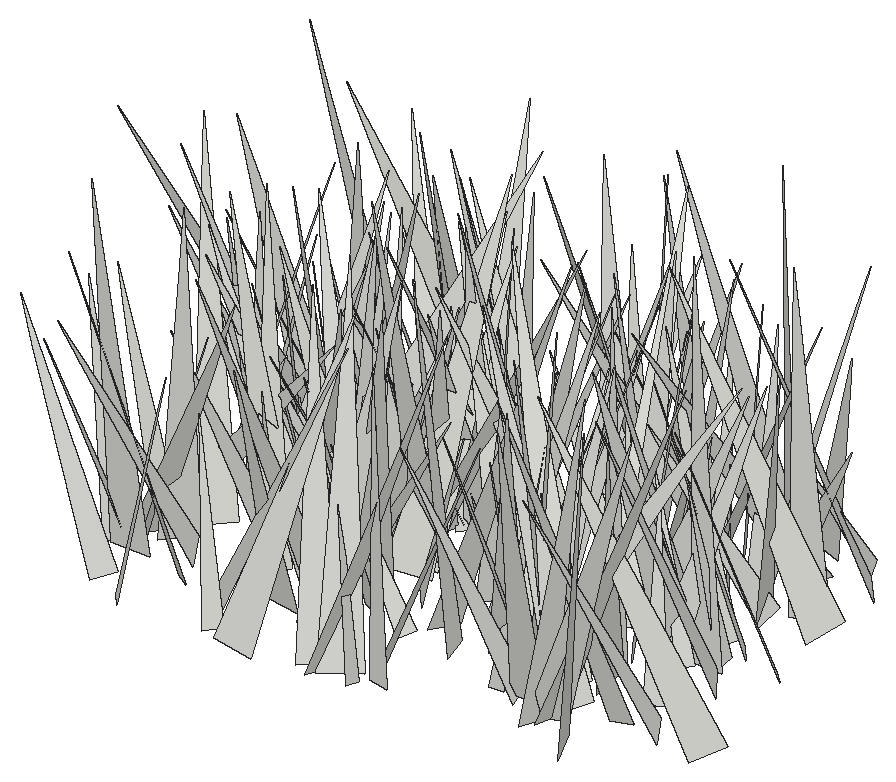
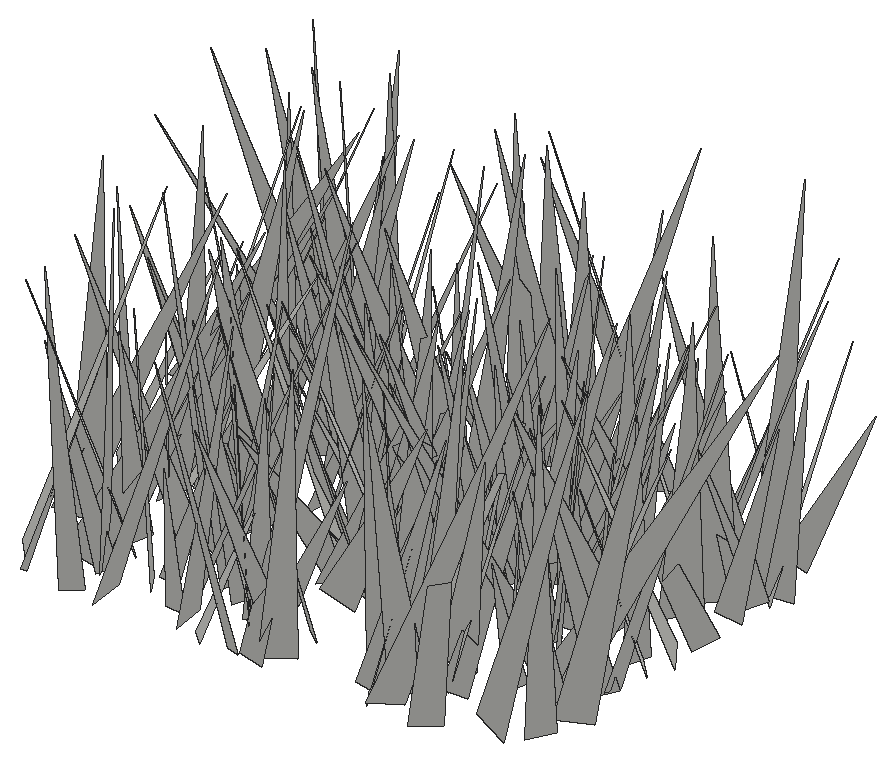
# SketchUp Ruby script. Lengths in inches.
U = 1.inch
M = Sketchup.active_model
def pt(a) = Geom::Point3d.new(a.map { |v| v * U })
def face(e, loops, mat)
  f = e.add_face(loops[0].map { |a| pt(a) })
  loops[1..].each { |l| e.add_face(l.map { |a| pt(a) }).erase! }
  f.material = f.back_material = mat if mat
  f
end
# faces: each face lists its corners as indices into pts; further lists are holes
def faces(e, pts, list, mat = nil) = list.each { |f| face(e, (f[0].is_a?(Array) ? f : [f]).map { |l| l.map { |i| pts[i] } }, mat) }
# xy, xz, yz: faces in a plane at the given z, y or x. An outline is a flat list of corners, or four numbers for a rectangle; further outlines are holes
def ring(l) = l.size == 4 ? [[l[0], l[1]], [l[2], l[1]], [l[2], l[3]], [l[0], l[3]]] : l.each_slice(2).to_a
def flat(e, list, mat, &to3) = list.each { |f| face(e, (f[0].is_a?(Array) ? f : [f]).map { |l| ring(l).map { |u, v| to3.(u, v) } }, mat) }
def xy(e, z, list, mat = nil) = flat(e, list, mat) { |x, y| [x, y, z] }
def xz(e, y, list, mat = nil) = flat(e, list, mat) { |x, z| [x, y, z] }
def yz(e, x, list, mat = nil) = flat(e, list, mat) { |y, z| [x, y, z] }
def lines(e, pts, list) = list.each { |a, b| e.add_line(pt(pts[a]), pt(pts[b])) }
# prism: a flat outline (further loops are holes) pulled along v
def prism(e, loops, v, mat = nil)
  f = face(e, loops, mat); d = Geom::Vector3d.new(v.map { |x| x * U })
  f.pushpull(f.normal.samedirection?(d) ? d.length : -d.length)
end
def box(e, o, s, mat = nil) = prism(e, [[o, [o[0] + s[0], o[1], o[2]], [o[0] + s[0], o[1] + s[1], o[2]], [o[0], o[1] + s[1], o[2]]]], [0, 0, s[2]], mat)
def at(x, y, z, deg = 0) = Geom::Transformation.translation(pt([x, y, z])) * Geom::Transformation.rotation(ORIGIN, Z_AXIS, deg.degrees)
def axes(o, x, y, z) = Geom::Transformation.new([*x, 0, *y, 0, *z, 0, *pt(o).to_a, 1])
def part(name) = M.definitions.add(name)
# library, detail: a bought-in or finely detailed component or shape, given as its bounding box
def library(name, o, s) = part(name).tap { |d| box(d.entities, o, s) }
def detail(e, o, s) = box(e.add_group.entities, o, s)
def put(e, d, t, mat = nil) = e.add_instance(d, t).tap { |i| i.material = mat if mat }
def group(e, t, mat = nil) = e.add_group.tap { |g| g.transformation = t; g.material = mat if mat }.entities
root = M.entities
c1 = part("fur_instance\#9")
p = [[0.8125,0,1.79],[0.67,-0.02,1.48],[0,-0.11,0],[0,0.11,0]]
faces(c1.entities,p,[[0,1,2,3]])
put(root,c1,axes([86.82,379.27,-27.1],[6.37942,2.61315,2.43113],[3.05762,-6.56979,-0.96169],[-1.84118,-1.85616,6.82648]))
put(root,c1,axes([67.4,377.72,-27.1],[3.19373,2.97376,0.94617],[2.91746,-3.32577,0.60507],[-1.10768,-0.18543,4.3217]))
put(root,c1,axes([71.48,378.1875,-27.1],[-3.55756,1.9012,0.49829],[1.88183,3.59228,-0.2708],[0.56709,0.00632,4.02461]))
put(root,c1,axes([72.91,377.54,-27.1],[-0.40245,7.17423,1.83924],[7.10701,0.89237,-1.92572],[2.08393,-1.65784,6.92265]))
put(root,c1,axes([70.46,379.66,-27.1],[6.41393,4.45568,0.74677],[4.39818,-5.86174,-2.80093],[1.0328,-2.70854,7.29015]))
put(root,c1,axes([83.7,381.16,-27.1],[0.50064,-7.21064,0.91051],[-7.21991,-0.3887,0.89157],[0.83387,0.96363,7.17281]))
put(root,c1,axes([77.92,378.21,-27.1],[-4.02809,-0.22088,0.67447],[-0.39433,3.92835,-1.06856],[0.59008,1.11738,3.89005]))
put(root,c1,axes([72.41,381.13,-27.1],[-0.34138,-6.1128,0.75859],[-6.1403,0.39794,0.44341],[0.48829,0.7305,6.10625]))
put(root,c1,axes([67.4,382.32,-27.1],[-5.6995,-3.45113,0.56108],[-3.05969,5.44221,2.39374],[1.69215,-1.78365,6.21808]))
put(root,c1,axes([74.41,381.4375,-27.1],[-0.98604,-7.77609,1.14314],[-7.75331,0.77346,-1.42635],[-1.28859,1.29646,7.70749]))
put(root,c1,axes([78.7,378.72,-27.1],[2.01081,5.29668,2.07869],[5.40677,-2.46554,1.0522],[-1.77275,-1.51176,5.56697]))
put(root,c1,axes([64.83,381.62,-27.1],[-3.71629,-3.62879,0.54604],[-3.4741,3.72939,1.13989],[1.18191,-0.44788,5.0675]))
put(root,c1,axes([65.96,378.8,-27.1],[-1.87407,5.07403,0.37598],[4.58214,1.50899,2.47512],[-2.21159,-1.17322,4.80954]))
put(root,c1,axes([83.11,381.43,-27.1],[-5.60277,-1.40853,0.55452],[-1.25772,5.51462,1.29985],[0.84237,-1.13469,5.62898]))
put(root,c1,axes([88.72,382.41,-27.1],[-5.31145,-3.30369,0.30508],[-3.10318,5.15062,1.7494],[1.17379,-1.33255,6.00546]))
put(root,c1,axes([76.02,378.6,-27.1],[-5.00326,5.02156,1.24961],[5.08502,5.09325,-0.10752],[0.95924,-0.80806,7.08781]))
put(root,c1,axes([65.47,380.93,-27.1],[-0.06707,-7.91469,2.47451],[-8.29222,0.04381,-0.08466],[-0.06773,2.47503,7.91452]))
put(root,c1,axes([76.33,378.13,-27.1],[6.99612,0.8962,1.32294],[0.53893,-6.91662,1.83548],[-1.5043,1.69005,6.81028]))
put(root,c1,axes([77.11,378.53,-27.1],[-4.81371,6.17541,1.55135],[6.27572,4.93015,-0.15223],[1.07597,-1.1279,7.82843]))
put(root,c1,axes([68.33,380.37,-27.1],[-4.54723,-4.75664,0.92618],[-4.80738,4.26788,-1.68375],[-0.61038,1.82216,6.36144]))
put(root,c1,axes([85.05,380.57,-27.1],[5.41416,-4.66063,0.97473],[-4.76032,-5.26587,1.26282],[0.1044,1.59183,7.03135]))
put(root,c1,axes([84.84,380.18,-27.1],[6.67765,-1.57713,2.05629],[-1.75682,-6.93326,0.38749],[-1.90506,0.86558,6.85042]))
put(root,c1,axes([81.29,383.01,-27.1],[1.38948,-7.3294,0.52561],[-7.22169,-1.26322,1.47599],[1.35779,0.7818,7.31247]))
put(root,c1,axes([82.22,383.17,-27.1],[-4.28945,-4.51982,0.83876],[-4.25056,4.33652,1.63064],[1.75072,-0.54543,6.01408]))
put(root,c1,axes([74.53,380.42,-27.1],[-0.74897,7.24815,2.93985],[7.55595,1.43371,-1.60981],[2.0214,-2.6736,7.1067]))
put(root,c1,axes([87.3,382.05,-27.1],[-2.01567,-6.30283,1.43527],[-6.28052,1.55369,-1.99742],[-1.52993,1.92587,6.30864]))
put(root,c1,axes([75.15,382.85,-27.1],[-2.33347,-4.94017,0.88075],[-4.99474,2.38012,0.11709],[0.48332,0.74554,5.4623]))
put(root,c1,axes([64.7,381.16,-27.1],[-2.06507,4.56305,1.47225],[4.79287,1.92061,0.77009],[-0.13147,-1.65628,4.94903]))
put(root,c1,axes([85.13,380.65,-27.1],[7.79072,-0.23447,0.87822],[-0.35324,-7.76347,1.06082],[-0.83754,1.09323,7.72172]))
put(root,c1,axes([72.3125,383.0625,-27.1],[-4.28655,1.17606,1.86698],[1.8295,4.17484,1.57066],[1.23356,-2.10497,4.15821]))
put(root,c1,axes([74.13,383.9,-27.1],[5.44226,-5.9088,0.26751],[-5.91243,-5.44486,0.01623],[-0.16928,0.20777,8.03317]))
put(root,c1,axes([91.21,382.15,-27.1],[-4.16636,5.9481,1.52453],[5.74666,3.12806,3.50054],[-2.16332,-3.14611,6.36276]))
put(root,c1,axes([65.1,382.26,-27.1],[5.86888,-2.59714,0.14419],[-2.59865,-5.83866,0.60558],[0.11385,0.61201,6.38922]))
put(root,c1,axes([85.16,384.0625,-27.1],[6.59264,-0.88288,1.14982],[-0.53637,-6.4595,-1.88457],[-1.3468,-1.74924,6.37893]))
put(root,c1,axes([85.06,381.23,-27.1],[-4.32916,0.66549,1.27706],[0.40908,4.44763,-0.93094],[1.38073,0.76884,4.27993]))
put(root,c1,axes([66.33,382.7,-27.1],[-4.86484,4.13925,3.64162],[4.78109,5.5858,0.03796],[2.74517,-2.39309,6.38738]))
put(root,c1,axes([84.28,381.98,-27.1],[-5.98871,-2.33617,1.80164],[-2.60473,6.10133,-0.74665],[1.38529,1.37273,6.38474]))
put(root,c1,axes([77.84,380.1,-27.1],[3.89032,1.8987,0.46131],[1.51623,-3.58179,1.95558],[-1.23244,1.58688,3.86204]))
put(root,c1,axes([85.3125,381.73,-27.1],[-7.32829,2.58062,0.59876],[2.60966,7.33524,0.32553],[0.45582,-0.50666,7.76257]))
put(root,c1,axes([82.47,382.88,-27.1],[5.33637,4.77614,2.80857],[5.34994,-5.45601,-0.88678],[-1.44141,-2.56842,7.10647]))
put(root,c1,axes([79.25,382.46,-27.1],[-6.68963,-2.36331,2.10659],[-2.62997,6.88987,-0.62215],[1.76244,1.31094,7.06748]))
put(root,c1,axes([89.59,383.45,-27.1],[-6.11827,1.22354,0.04324],[1.20265,5.96505,1.37981],[-0.22923,-1.36132,6.08493]))
put(root,c1,axes([77.21,382.24,-27.1],[-1.66623,3.3763,0.05798],[2.90925,1.40249,1.93607],[-1.71436,-0.9015,3.22914]))
put(root,c1,axes([65.49,381.56,-27.1],[3.79033,1.52401,0.8214],[1.29616,-3.80865,1.0854],[-1.14773,0.73179,3.93842]))
put(root,c1,axes([81.27,383.68,-27.1],[-2.39364,-3.13142,1.17859],[-3.27618,2.48779,-0.04385],[0.67935,0.9641,3.94124]))
put(root,c1,axes([68.75,384.91,-27.1],[0.69444,-4.60057,1.02449],[-4.36557,-1.0182,-1.61314],[-1.77671,0.70364,4.36409]))
put(root,c1,axes([82.21,381.15,-27.1],[2.45384,5.3856,0.3895],[5.06414,-2.44383,1.88676],[-1.87372,0.44803,5.60947]))
put(root,c1,axes([83.4375,383.82,-27.1],[-3.37227,-0.8607,0.92289],[-0.91034,3.4828,-0.07828],[0.87397,0.30665,3.4795]))
put(root,c1,axes([88.16,386.44,-27.1],[-5.39374,-4.42373,0.73063],[-4.15874,5.36317,1.77113],[1.67573,-0.92879,6.74722]))
put(root,c1,axes([75.81,384.79,-27.1],[3.73133,2.74864,1.27928],[3.02044,-3.19509,-1.94493],[0.26177,-2.31318,4.20655]))
put(root,c1,axes([65.27,383.4,-27.1],[-1.60239,4.56784,1.22355],[4.62571,1.24567,1.40748],[-0.98238,-1.58525,4.63161]))
put(root,c1,axes([69.11,384.76,-27.1],[3.4639,-0.21189,1.20284],[0.06017,-3.58323,-0.80448],[-1.21988,-0.7784,3.37584]))
put(root,c1,axes([70.13,383.94,-27.1],[-6.35948,3.06032,1.72749],[3.24757,6.48259,0.47123],[1.34279,-1.18457,7.04176]))
put(root,c1,axes([82.43,382.77,-27.1],[3.56611,7.00423,0.23479],[6.50816,-3.2121,-3.02618],[2.59966,-1.56674,7.25387]))
put(root,c1,axes([87.46,383.78,-27.1],[-1.55614,3.71904,0.91385],[3.82438,1.56093,0.15988],[0.20123,-0.90564,4.0283]))
put(root,c1,axes([70.16,383.97,-27.1],[-2.19401,4.08598,0.64459],[3.98986,1.89782,1.55038],[-1.09165,-1.27572,4.37096]))
put(root,c1,axes([73.15,384.03,-27.1],[4.12414,-1.44643,0.07491],[-1.4095,-3.95608,1.21201],[0.33327,1.1677,4.19901]))
put(root,c1,axes([84,383.02,-27.1],[-6.13421,5.52562,0.24546],[5.52788,6.11218,0.5523],[-0.18784,-0.57446,8.23747]))
put(root,c1,axes([70.47,382.9,-27.1],[-6.55915,2.85076,0.80174],[2.70921,6.56329,-1.17278],[1.19574,0.76707,7.05506]))
put(root,c1,axes([82.21,383.78,-27.1],[-0.35457,5.93898,1.63328],[6.05839,0.63143,-0.98081],[1.11129,-1.54746,5.86815]))
put(root,c1,axes([73.56,386,-27.1],[-2.21504,-4.22644,0.02495],[-4.06696,2.12371,-1.31133],[-1.15036,0.62998,4.58799]))
put(root,c1,axes([64.6875,385.44,-27.1],[2.58062,-5.27777,0.62862],[-4.46822,-1.77579,3.43383],[2.87837,1.97518,4.76689]))
put(root,c1,axes([69.66,386.86,-27.1],[6.23542,-1.61716,0.46655],[-1.48447,-6.12774,-1.40019],[-0.79324,-1.24458,6.2877]))
put(root,c1,axes([85.625,387.6,-27.1],[5.45366,-4.66647,1.60556],[-4.21255,-5.64853,-2.10822],[-2.57063,-0.64365,6.86103]))
put(root,c1,axes([70.11,385.39,-27.1],[-5.34119,3.3335,0.99515],[3.47843,5.14626,1.43085],[0.05516,-1.74201,6.13133]))
put(root,c1,axes([79.4375,384.82,-27.1],[2.86437,6.58912,2.04567],[6.83224,-2.40073,-1.83379],[0.96006,-2.57407,6.94682]))
put(root,c1,axes([77.86,383.58,-27.1],[7.57177,-0.43303,1.80554],[-0.88332,-7.50835,1.90355],[-1.63317,2.05334,7.34137]))
put(root,c1,axes([81.09,383.83,-27.1],[-3.67286,3.55796,0.5072],[3.52102,3.70767,-0.51167],[0.72023,0.01818,5.08794]))
put(root,c1,axes([74.72,386.87,-27.1],[-1.19832,-8.06423,2.00487],[-8.30399,1.23724,0.01324],[0.30817,1.98109,8.15276]))
put(root,c1,axes([78.06,386.12,-27.1],[3.7544,-3.60472,1.46029],[-3.77286,-3.86843,0.15082],[-0.94444,1.12393,5.20257]))
put(root,c1,axes([84.68,385,-27.1],[1.78909,6.44129,2.50482],[6.73985,-2.19865,0.83993],[-1.52927,-2.15428,6.63216]))
put(root,c1,axes([72.03,386.16,-27.1],[-5.02266,3.34128,1.54054],[3.64584,4.87057,1.32283],[0.49523,-1.96924,5.88569]))
put(root,c1,axes([69.45,387.61,-27.1],[3.15853,-4.87453,2.05329],[-4.28659,-3.76007,-2.33247],[-3.09874,0.23284,5.31949]))
put(root,c1,axes([66.7,384.33,-27.1],[-6.24341,4.5177,1.05822],[4.50521,6.32678,-0.4296],[1.11019,-0.26807,7.69449]))
put(root,c1,axes([69.52,386.68,-27.1],[-3.89073,-3.2521,0.98713],[-3.3181,3.95947,-0.03367],[0.73538,0.65937,5.07078]))
put(root,c1,axes([72.9,385.89,-27.1],[4.30722,-1.10997,0.82887],[-1.21703,-4.32511,0.53238],[-0.66174,0.72977,4.41597]))
put(root,c1,axes([70.14,386.71,-27.1],[-7.66892,-1.90839,0.15613],[-1.91216,7.66661,-0.21311],[0.09999,0.24454,7.89993]))
put(root,c1,axes([66.61,387.25,-27.1],[-5.67591,-0.59927,2.29984],[-0.30227,6.08824,0.84044],[2.35734,-0.66225,5.64524]))
put(root,c1,axes([81.92,386.47,-27.1],[-5.15429,0.32159,0.0951],[0.32057,5.15491,-0.05731],[0.09848,0.05128,5.164]))
put(root,c1,axes([80.93,387,-27.1],[-7.3033,-3.33888,1.09507],[-3.45877,7.27632,-0.88176],[0.61989,1.26191,7.98178]))
put(root,c1,axes([69.2,388.52,-27.1],[6.14406,2.36607,3.59044],[3.36505,-6.54408,-1.44586],[-2.67694,-2.79567,6.42319]))
put(root,c1,axes([73.43,388.87,-27.1],[5.23311,-3.59302,0.50013],[-3.53385,-5.24745,-0.7222],[-0.81967,-0.31597,6.30664]))
put(root,c1,axes([71.98,385.66,-27.1],[-5.31881,4.24046,0.31909],[4.24772,5.322,0.07866],[0.20039,-0.26047,6.80184]))
put(root,c1,axes([72.93,384.17,-27.1],[1.87355,6.48838,0.26131],[6.01197,-1.83596,2.48253],[-2.45429,0.45575,6.28063]))
put(root,c1,axes([87.48,387.77,-27.1],[-3.67755,-0.2078,1.11626],[-0.0694,3.8179,0.48208],[1.13331,-0.4405,3.65173]))
put(root,c1,axes([71.16,386.72,-27.1],[1.59622,5.71911,2.00108],[6.0184,-1.73595,0.16062],[-0.70101,-1.88115,5.93551]))
put(root,c1,axes([84.43,386.23,-27.1],[5.20843,4.28763,1.83578],[4.29945,-5.48037,0.60158],[-1.80791,-0.68076,6.71935]))
put(root,c1,axes([89.64,388.16,-27.1],[-3.75562,-3.58045,0.3486],[-3.58145,3.67402,-0.84892],[-0.33818,0.85312,5.11895]))
put(root,c1,axes([65.1875,390.17,-27.1],[-6.16239,-2.08969,1.53365],[-1.42213,6.03269,2.50561],[2.16712,-1.98337,6.00531]))
put(root,c1,axes([79.35,385.98,-27.1],[3.38601,2.0667,0.33408],[1.88033,-3.28152,1.24252],[-0.92044,0.89903,3.76728]))
put(root,c1,axes([86.52,386.68,-27.1],[-0.98772,3.5916,0.11089],[3.35733,0.88143,1.35606],[-1.28071,-0.45933,3.46934]))
put(root,c1,axes([74.43,385.77,-27.1],[-3.17908,7.18759,1.82609],[7.05927,3.54175,-1.65087],[2.27218,-0.9472,7.68392]))
put(root,c1,axes([87.15,387.12,-27.1],[1.25442,7.48082,2.76942],[7.81491,-1.71475,1.09211],[-1.59984,-2.51056,7.50623]))
put(root,c1,axes([72.58,387.64,-27.1],[4.97792,-1.2009,1.19397],[-1.36113,-5.04298,0.6026],[-1.0075,0.87956,5.08515]))
put(root,c1,axes([85.42,387,-27.1],[0.44188,5.84269,1.52194],[5.83939,-0.02571,-1.59672],[1.53457,-1.58458,5.63763]))
put(root,c1,axes([74.9,389.9375,-27.1],[1.62052,-5.44249,0.65001],[-5.43307,-1.68456,-0.55967],[-0.72449,0.45919,5.65098]))
put(root,c1,axes([87.62,388.77,-27.1],[-4.41159,-3.54695,0.73212],[-3.61607,4.3782,-0.57829],[0.20221,0.91078,5.63104]))
put(root,c1,axes([73.36,385.91,-27.1],[1.09357,6.43106,0.77169],[6.11568,-1.28298,2.02542],[-2.13365,-0.38127,6.20097]))
put(root,c1,axes([72.23,389.6,-27.1],[-3.11173,-3.4795,0.92655],[-3.33661,3.24675,0.98692],[1.3537,0.0043,4.56244]))
put(root,c1,axes([65.85,387.97,-27.1],[-4.75498,1.70819,1.94206],[1.76287,5.11453,-0.18234],[1.89256,-0.47231,5.04921]))
put(root,c1,axes([73.33,390.19,-27.1],[-3.18461,-4.17271,0.10236],[-4.17132,3.18622,0.10881],[0.1486,0.01532,5.24799]))
put(root,c1,axes([75.9,390.62,-27.1],[-1.54524,-6.7658,0.51217],[-6.71547,1.44992,-1.10738],[-0.96994,0.74015,6.85109]))
put(root,c1,axes([77.31,388.77,-27.1],[6.16664,-2.56617,1.31423],[-2.70082,-6.22755,0.51287],[-1.00896,0.98602,6.65955]))
put(root,c1,axes([69.11,389.09,-27.1],[7.358,-0.55238,1.16955],[-0.51092,-7.44716,-0.30295],[-1.18825,-0.21839,7.37248]))
put(root,c1,axes([73.91,387.28,-27.1],[7.28902,-0.71217,0.57332],[-0.83779,-7.04721,1.89755],[-0.36604,1.94818,7.07364]))
put(root,c1,axes([67.05,390.84,-27.1],[-1.39061,-8.04384,0.83594],[-7.45661,0.94696,-3.29214],[-3.13068,1.31752,7.46987]))
put(root,c1,axes([74.43,386.53,-27.1],[-1.14169,6.19263,0.48775],[6.13199,1.20279,-0.91762],[0.99261,-0.30768,6.22978]))
put(root,c1,axes([67.7,390.29,-27.1],[-3.39488,-3.98848,1.56761],[-3.7052,3.73666,1.48306],[2.15333,0.14147,5.02331]))
put(root,c1,axes([66.82,389.33,-27.1],[-2.76326,-3.0585,1.38467],[-3.15346,2.97986,0.28892],[1.15213,0.82059,4.11176]))
put(root,c1,axes([86.87,387.49,-27.1],[-6.97142,-3.26118,0.0354],[-2.96258,6.29742,-3.28677],[-1.3637,2.99072,6.9594]))
put(root,c1,axes([78.18,390.34,-27.1],[-6.07615,0.58264,0.90457],[0.83184,5.83413,1.82981],[0.68247,-1.92372,5.8233]))
put(root,c1,axes([77.59,387.75,-27.1],[-3.01404,5.97197,0.86388],[5.95256,2.78442,1.51964],[-0.98886,-1.44144,6.51457]))
put(root,c1,axes([65,386.75,-27.1],[5.18703,3.91751,0.7095],[3.72248,-5.18551,1.41748],[-1.41191,0.72053,6.34373]))
put(root,c1,axes([74.58,390.03,-27.1],[2.81734,-6.20209,1.85033],[-6.41792,-2.93797,-0.07572],[-0.83667,1.65211,6.81158]))
put(root,c1,axes([77.36,390.13,-27.1],[-4.25466,-1.2014,1.34721],[-0.93808,4.41863,0.97784],[1.54219,-0.62673,4.31153]))
put(root,c1,axes([76.05,389.45,-27.1],[-1.30466,-3.28465,1.2487],[-3.51229,1.2605,-0.354],[0.10971,1.29326,3.5165]))
put(root,c1,axes([77.03,387.84,-27.1],[4.58247,4.01128,0.43645],[4.00699,-4.60163,0.22113],[-0.47421,-0.12046,6.08609]))
put(root,c1,axes([79.41,387.74,-27.1],[-0.73079,4.32054,0.1844],[4.30671,0.74406,-0.36572],[0.39156,-0.12013,4.36662]))
put(root,c1,axes([86.65,391.39,-27.1],[-4.86866,0.51762,1.11395],[0.97098,4.41082,2.19421],[0.75234,-2.34296,4.3769]))
put(root,c1,axes([78.57,388.875,-27.1],[5.68273,3.19615,0.64935],[3.24559,-5.67036,-0.49352],[-0.32122,-0.74969,6.50117]))
put(root,c1,axes([82.98,389.33,-27.1],[2.29321,-4.71361,1.70331],[-4.8602,-1.63403,2.02152],[1.22385,2.34308,4.83635]))
put(root,c1,axes([67.81,386.84,-27.1],[-5.19171,3.73852,1.55221],[3.028,5.26206,-2.54592],[2.68647,1.29382,5.8693]))
put(root,c1,axes([86.6,388.86,-27.1],[-5.80582,1.67481,0.45332],[1.66732,5.82342,-0.1609],[0.48013,0.02943,6.04042]))
put(root,c1,axes([75.09,389.45,-27.1],[-3.69691,-1.68274,0.52652],[-1.75981,3.59718,-0.85985],[0.10916,1.00233,3.96981]))
put(root,c1,axes([65.32,388.14,-27.1],[3.04107,3.48011,0.59696],[3.3547,-3.09349,0.94446],[-1.10161,0.1866,4.52408]))
put(root,c1,axes([65.24,390.52,-27.1],[2.87453,-4.20489,0.68169],[-4.14129,-2.56592,1.63539],[0.99777,1.46412,4.82385]))
put(root,c1,axes([86.32,391.51,-27.1],[6.10646,0.88523,1.50787],[1.27518,-6.00248,-1.64024],[-1.19633,-1.87958,5.94829]))
put(root,c1,axes([82.58,388.76,-27.1],[-5.70861,3.53079,2.01517],[3.32922,6.05385,-1.17592],[2.33318,0.00055,6.60847]))
put(root,c1,axes([68.99,391.07,-27.1],[-4.42725,-2.60663,1.07476],[-2.66002,4.52485,0.01676],[0.93485,0.53053,5.13759]))
put(root,c1,axes([74.09,389.63,-27.1],[-3.60805,2.068,0.36238],[2.05277,3.62596,-0.25393],[0.44056,0.04128,4.15092]))
put(root,c1,axes([66.03,392.33,-27.1],[-3.26059,-4.43586,0.10579],[-4.43536,3.26207,0.0775],[0.12511,0.03932,5.50476]))
put(root,c1,axes([82.9,389.68,-27.1],[-6.0397,-1.24718,1.08354],[-1.47294,5.92489,-1.39057],[0.74831,1.59618,6.00831]))
put(root,c1,axes([69.53,393.93,-27.1],[4.70734,-3.12135,0.14145],[-2.64852,-4.12178,-2.81392],[-1.65776,-2.27815,4.89732]))
put(root,c1,axes([72.9,388.29,-27.1],[-1.71935,6.00909,0.23442],[5.94835,1.73522,-0.85232],[0.8839,0.01135,6.19184]))
put(root,c1,axes([88.93,391.78,-27.1],[-7.28796,2.50197,0.93453],[2.66483,6.99355,2.0583],[0.17855,-2.25345,7.42547]))
put(root,c1,axes([82.76,387.55,-27.1],[-4.41357,6.91206,0.00056],[6.86097,4.38103,-0.99489],[0.83882,0.53496,8.14041]))
put(root,c1,axes([82.66,391.3,-27.1],[-2.78435,-5.66723,3.39056],[-5.97834,3.72634,1.319],[2.80584,2.3158,6.17497]))
put(root,c1,axes([75.77,390.88,-27.1],[4.35224,4.23695,0.82253],[4.28263,-4.09432,-1.57033],[0.53605,-1.68972,5.86752]))
put(root,c1,axes([64.83,392.85,-27.1],[4.91943,-4.73173,2.30235],[-4.40019,-5.42749,-1.75256],[-2.8859,0.2095,6.59686]))
put(root,c1,axes([86.2,394.54,-27.1],[2.18391,-6.70079,0.42323],[-6.08063,-2.16263,-2.86325],[-2.84706,-0.52116,6.43986]))
put(root,c1,axes([84.6,391.5625,-27.1],[2.87799,2.64757,1.74089],[2.94858,-3.09885,-0.16173],[-1.16026,-1.30792,3.90721]))
put(root,c1,axes([80.87,394.9375,-27.1],[-6.78403,-3.28205,0.63683],[-2.89291,6.48484,2.60352],[1.67585,-2.09175,7.07224]))
put(root,c1,axes([87.93,392.14,-27.1],[1.68119,-6.78383,2.85706],[-7.30642,-1.89388,-0.19753],[-0.89411,2.72073,6.98625]))
put(root,c1,axes([83.46,391.49,-27.1],[6.47298,0.85818,0.33872],[0.84258,-6.4766,0.30739],[-0.37587,0.26066,6.52238]))
put(root,c1,axes([67.67,393.18,-27.1],[3.15596,1.30372,1.61225],[1.82364,-3.14251,-1.02861],[-0.98659,-1.6383,3.25603]))
put(root,c1,axes([80.8125,392.86,-27.1],[3.7872,-0.0255,0.26622],[0.02172,-3.73751,-0.66706],[-0.26655,-0.66693,3.72808]))
put(root,c1,axes([70.03,393.65,-27.1],[-3.79874,-3.55526,0.6962],[-3.51199,3.8615,0.55657],[0.88909,0.06302,5.17306]))
put(root,c1,axes([79.05,388.97,-27.1],[-4.90566,2.32822,0.51514],[1.6552,4.17303,-3.098],[1.71648,2.62995,4.45965]))
put(root,c1,axes([68.17,390.375,-27.1],[0.84349,7.5995,0.98427],[7.14395,-0.42161,-2.86687],[2.77222,-1.22577,7.08837]))
put(root,c1,axes([82.73,393.87,-27.1],[0.53786,-3.60504,0.14249],[-3.55289,-0.5543,-0.6129],[-0.62738,0.04841,3.59304]))
put(root,c1,axes([78.45,392.29,-27.1],[-1.80359,3.13263,0.44398],[3.00697,1.53819,1.36218],[-0.98418,-1.04117,3.34825]))
put(root,c1,axes([73.66,391.81,-27.1],[0.00503,4.167,0.7042],[4.17874,-0.11,0.62111],[-0.63075,-0.69557,4.12045]))
put(root,c1,axes([72.98,392.79,-27.1],[4.34542,2.75412,2.00138],[2.98226,-4.64462,-0.0836],[-1.6422,-1.14703,5.14401]))
put(root,c1,axes([77.11,391.17,-27.1],[-1.95645,6.57203,0.15793],[5.85701,1.66776,3.15567],[-2.98529,-1.03499,6.08778]))
put(root,c1,axes([79.6875,393.24,-27.1],[5.0608,-1.8582,0.79428],[-1.91101,-5.09708,0.2516],[-0.65714,0.51221,5.38529]))
put(root,c1,axes([78.59,394.21,-27.1],[4.23217,0.79223,1.75299],[1.35483,-4.23497,-1.35698],[-1.36567,-1.74623,4.08626]))
put(root,c1,axes([69.9375,394.875,-27.1],[-3.5221,-6.63629,1.77015],[-6.5539,3.84233,1.36448],[2.0543,0.8804,7.38808]))
put(root,c1,axes([66.11,392.15,-27.1],[0.58745,4.61701,1.14714],[4.75417,-0.52722,-0.31264],[0.17496,-1.17604,4.64372]))
put(root,c1,axes([88.25,395.33,-27.1],[-5.65228,-5.31186,0.60473],[-5.29476,5.68375,0.43618],[0.73959,0.09466,7.74428]))
put(root,c1,axes([85.47,392.18,-27.1],[-4.49774,2.41965,1.22715],[2.26445,4.65664,-0.88215],[1.49428,0.22634,5.03052]))
put(root,c1,axes([65.13,394.39,-27.1],[5.79339,-2.08626,1.56673],[-1.97661,-6.00002,-0.68061],[-1.70297,-0.13319,6.11985]))
put(root,c1,axes([76.8,396.55,-27.1],[-3.41876,-7.6362,0.72671],[-7.48826,3.49493,1.49637],[1.66304,0.03883,8.23167]))
put(root,c1,axes([84.99,394.63,-27.1],[1.43751,-4.12245,0.23292],[-3.7226,-1.18725,1.96162],[1.78636,0.84328,3.90039]))
put(root,c1,axes([71,396.04,-27.1],[-7.92224,1.63819,2.17065],[2.33717,7.51957,2.85498],[1.39032,-3.306,7.56932]))
put(root,c1,axes([68.85,396.39,-27.1],[6.56004,-2.8558,0.90961],[-2.50702,-6.42798,-2.10074],[-1.6425,-1.59457,6.83935]))
put(root,c1,axes([68.02,392.2,-27.1],[-3.33951,2.40161,0.05247],[2.31618,3.24301,-1.02031],[0.63702,0.79874,3.98485]))
put(root,c1,axes([72.96,393.85,-27.1],[5.47635,-0.94494,2.24683],[-1.1073,-5.8869,0.22307],[-2.17142,0.61884,5.55279]))
put(root,c1,axes([76.0625,393.84,-27.1],[4.67492,4.49227,1.13099],[4.6277,-4.45606,-1.42912],[0.20972,-1.8104,6.324]))
put(root,c1,axes([70.71,392.2,-27.1],[-2.20757,6.36235,0.08993],[6.1827,2.12231,1.62203],[-1.50393,-0.61421,6.5362]))
put(root,c1,axes([83.06,394.42,-27.1],[4.36466,2.86173,1.95624],[3.18404,-4.55325,-0.44325],[-1.3705,-1.46462,5.20032]))
put(root,c1,axes([87.36,396.49,-27.1],[-3.37323,-1.69913,0.74168],[-1.13548,3.11072,1.96213],[1.46554,-1.50074,3.22735]))
put(root,c1,axes([85.39,392.65,-27.1],[4.30738,5.01035,0.65824],[4.94004,-4.35705,0.83813],[-1.06435,0.05398,6.55397]))
put(root,c1,axes([66.9375,395.06,-27.1],[-2.69995,-7.06667,2.40673],[-7.39529,2.18224,-1.88876],[-1.01973,2.88442,7.32531]))
put(root,c1,axes([78.63,394.4375,-27.1],[-4.89725,-3.9807,3.26033],[-4.56553,5.43754,-0.21877],[2.37312,2.24631,6.30723]))
put(root,c1,axes([85.51,394.09,-27.1],[-6.98093,-2.98191,2.95578],[-3.56155,7.24267,-1.10492],[2.22346,2.23913,7.51028]))
put(root,c1,axes([78.3,394.26,-27.1],[-1.55203,4.86816,1.43833],[5.0761,1.479,0.47157],[-0.03172,-1.51332,5.08777]))
put(root,c1,axes([78.52,394.24,-27.1],[2.84043,2.51238,0.82611],[2.52394,-2.93724,0.2547],[-0.79009,-0.35083,3.78354]))
put(root,c1,axes([85.09,396.54,-27.1],[0.27487,-5.90315,0.86813],[-5.62576,0.03312,2.00651],[1.98787,0.91,5.55848]))
put(root,c1,axes([79.32,396.47,-27.1],[-2.85386,-2.94003,0.13695],[-2.93623,2.85714,0.14971],[0.2028,-0.00613,4.09462]))
put(root,c1,axes([72.04,395.59,-27.1],[-1.46223,5.38545,2.28823],[5.73287,0.84616,1.67196],[-1.17188,-2.58033,5.32407]))
put(root,c1,axes([83.88,396.09,-27.1],[-7.9003,-1.05971,0.99848],[-1.05239,7.96314,0.1246],[1.0062,0.00826,7.97008]))
put(root,c1,axes([71.79,396.02,-27.1],[-4.56615,-2.82263,0.99228],[-2.92894,4.58662,-0.43101],[0.61084,0.89289,5.35081]))
put(root,c1,axes([80.45,395.6,-27.1],[-6.61174,-0.50833,1.66504],[-0.62205,6.79727,-0.39495],[1.62598,0.53342,6.61948]))
put(root,c1,axes([76.11,395.85,-27.1],[-4.07853,4.6775,2.02917],[4.97181,4.22458,0.25488],[1.13033,-1.70436,6.20068]))
put(root,c1,axes([76.8125,394.8,-27.1],[-1.32926,4.80497,0.97182],[4.66035,1.55098,-1.29408],[1.52094,-0.553,4.81456]))
put(root,c1,axes([70.79,394.9375,-27.1],[-3.43213,5.64571,1.59286],[5.69776,3.64732,-0.65059],[1.39526,-1.00684,6.57497]))
put(root,c1,axes([81.24,395.39,-27.1],[-0.33834,3.74046,0.53618],[3.75079,0.26714,0.50319],[-0.45836,-0.57497,3.72187]))
put(root,c1,axes([77.7,396.47,-27.1],[3.43659,4.37627,1.35344],[4.55407,-3.08156,-1.59944],[0.49399,-2.03617,5.32951]))
